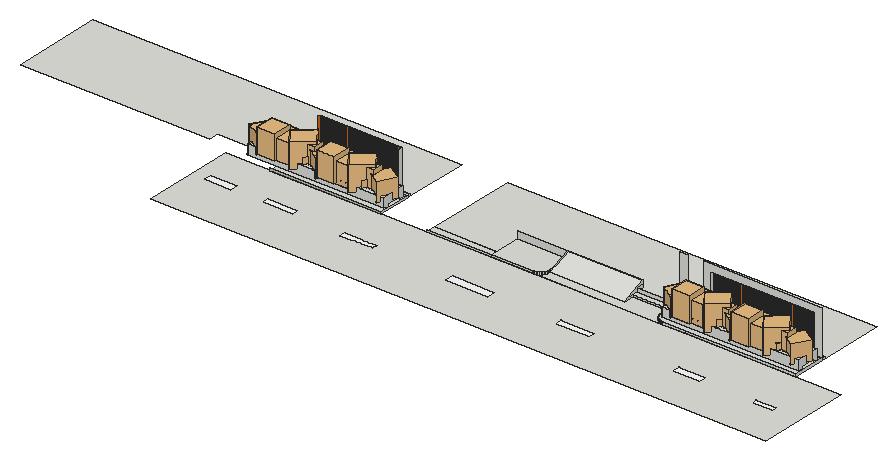
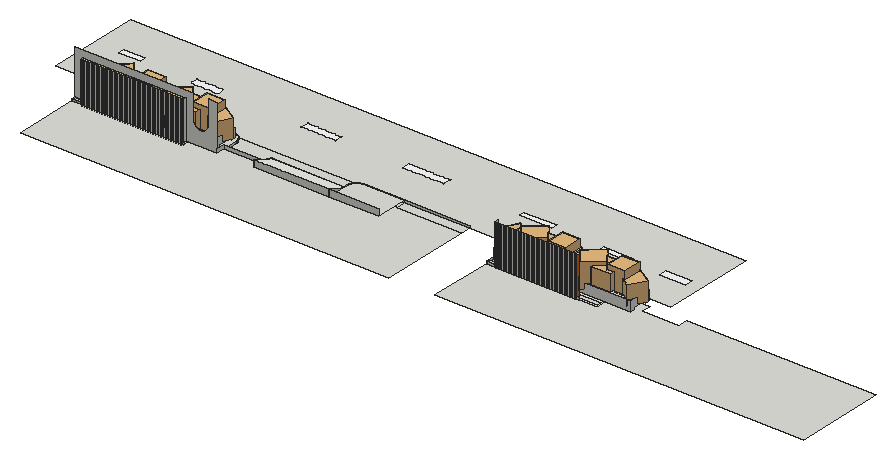
# SketchUp Ruby script. Lengths in inches.
U = 1.inch
M = Sketchup.active_model
def pt(a) = Geom::Point3d.new(a.map { |v| v * U })
def face(e, loops, mat)
  f = e.add_face(loops[0].map { |a| pt(a) })
  loops[1..].each { |l| e.add_face(l.map { |a| pt(a) }).erase! }
  f.material = f.back_material = mat if mat
  f
end
# faces: each face lists its corners as indices into pts; further lists are holes
def faces(e, pts, list, mat = nil) = list.each { |f| face(e, (f[0].is_a?(Array) ? f : [f]).map { |l| l.map { |i| pts[i] } }, mat) }
# xy, xz, yz: faces in a plane at the given z, y or x. An outline is a flat list of corners, or four numbers for a rectangle; further outlines are holes
def ring(l) = l.size == 4 ? [[l[0], l[1]], [l[2], l[1]], [l[2], l[3]], [l[0], l[3]]] : l.each_slice(2).to_a
def flat(e, list, mat, &to3) = list.each { |f| face(e, (f[0].is_a?(Array) ? f : [f]).map { |l| ring(l).map { |u, v| to3.(u, v) } }, mat) }
def xy(e, z, list, mat = nil) = flat(e, list, mat) { |x, y| [x, y, z] }
def xz(e, y, list, mat = nil) = flat(e, list, mat) { |x, z| [x, y, z] }
def yz(e, x, list, mat = nil) = flat(e, list, mat) { |y, z| [x, y, z] }
def lines(e, pts, list) = list.each { |a, b| e.add_line(pt(pts[a]), pt(pts[b])) }
# prism: a flat outline (further loops are holes) pulled along v
def prism(e, loops, v, mat = nil)
  f = face(e, loops, mat); d = Geom::Vector3d.new(v.map { |x| x * U })
  f.pushpull(f.normal.samedirection?(d) ? d.length : -d.length)
end
def box(e, o, s, mat = nil) = prism(e, [[o, [o[0] + s[0], o[1], o[2]], [o[0] + s[0], o[1] + s[1], o[2]], [o[0], o[1] + s[1], o[2]]]], [0, 0, s[2]], mat)
def at(x, y, z, deg = 0) = Geom::Transformation.translation(pt([x, y, z])) * Geom::Transformation.rotation(ORIGIN, Z_AXIS, deg.degrees)
def axes(o, x, y, z) = Geom::Transformation.new([*x, 0, *y, 0, *z, 0, *pt(o).to_a, 1])
def part(name) = M.definitions.add(name)
# library, detail: a bought-in or finely detailed component or shape, given as its bounding box
def library(name, o, s) = part(name).tap { |d| box(d.entities, o, s) }
def detail(e, o, s) = box(e.add_group.entities, o, s)
def put(e, d, t, mat = nil) = e.add_instance(d, t).tap { |i| i.material = mat if mat }
def group(e, t, mat = nil) = e.add_group.tap { |g| g.transformation = t; g.material = mat if mat }.entities
root = M.entities
M.materials.add("Color_000").color = [255, 255, 255]
M.materials.add("Material__1").color = [95, 70, 46]
M.materials.add("[0041_Chocolate]").color = [210, 105, 30]
M.materials.add("[Pavers with Grass Herringbone]").color = [197, 201, 190]
c1 = part("Untitled (5)")
xy(c1.entities,0,[[[158.81,26.5625,306.06,993.3125],[226.57,518.17,239.57,583.92],[225.28,357.51,237.28,411.51],[222.61,182.28,236.36,226.53],[239.71,931.55,251.46,972.3],[233.64,703.93,242.14,755.18],[240.05,835.03,248.8,880.53],[222.04,66.5,231.29,100.5]]])
xy(c1.entities,0,[[222.04,66.5,231.29,100.5],[222.61,182.28,236.36,226.53],[225.28,357.51,237.28,411.51],[226.57,518.17,239.57,583.92],[233.64,703.93,242.14,755.18],
  [240.05,835.03,248.8,880.53],[239.71,931.55,251.46,972.3]],"Color_000")
c2 = library("Areca palm plant",[0,0,0],[49.1,36.6,54.46])
c3 = library("Group\#74",[-84.69,-90.07,-0.36],[176.51,175.13,171.4])
c4 = library("Group20\#1",[-20.81,-17.08,3.79],[39.86,39.43,37.51])
c5 = library("Group38\#2",[14.01,28.44,-23.43],[18.58,18.32,38.89])
c6 = library("Group\#130",[-7.34,-1.2,0],[38.67,35.81,49.04])
c7 = part("Group\#8")
put(c7.entities,c2,axes([-6.2,56.6,6.08],[0.45017,-0.56191,0],[0.66137,0.52986,0],[0,0,0.72]))
put(c7.entities,c2,axes([-6.2,158.41,6.08],[0.45017,-0.56191,0],[0.66137,0.52986,0],[0,0,0.72]))
put(c7.entities,c3,axes([14.93,145.87,6.05],[-0.04961,-0.08593,0],[0.08593,-0.04961,0],[0,0,0.10522]))
put(c7.entities,c3,axes([14.93,193.18,6.05],[-0.04961,-0.08593,0],[0.08593,-0.04961,0],[0,0,0.10522]))
put(c7.entities,c4,axes([18.97,79.98,4.77],[0,0.85,0],[-0.85,0,0],[0,0,0.85]))
put(c7.entities,c3,axes([14.93,173.12,6.05],[-0.04961,-0.08593,0],[0.08593,-0.04961,0],[0,0,0.10522]))
g1 = group(c7.entities,at(0,0,0))
xy(g1,0,[[0,0,6,234.8],[30,0,36,234.8]])
xy(g1,3,[[6,0,30,234.8]])
xy(g1,7,[[6,5,30,229.8]],"Material__1")
xy(g1,15,[[[0,0,36,234.8],[6,5,30,229.8]]])
xz(g1,0,[[0,0,6,0,6,3,30,3,30,0,36,0,36,15,0,15]])
xz(g1,5,[[6,7,30,15]])
xz(g1,229.8,[[6,7,30,15]])
xz(g1,234.8,[[0,0,0,15,36,15,36,0,30,0,30,3,6,3,6,0]])
yz(g1,0,[[0,0,234.8,15]])
yz(g1,6,[[0,0,234.8,3],[5,7,229.8,15]])
yz(g1,30,[[0,0,234.8,3],[5,7,229.8,15]])
yz(g1,36,[[0,0,234.8,15]])
put(c7.entities,c3,axes([17.19,223.04,6.07],[-0.08133,-0.14087,0],[0.14087,-0.08133,0],[0,0,0.1725]))
put(c7.entities,c5,axes([-4.1,-1.15,28.17],[0.8848,0,0],[0,0.94674,0],[0,0,0.85826]))
put(c7.entities,c3,axes([17.19,15.79,6.07],[-0.08133,-0.14087,0],[0.14087,-0.08133,0],[0,0,0.1725]))
put(c7.entities,c3,axes([14.93,91.37,6.05],[-0.04961,-0.08593,0],[0.08593,-0.04961,0],[0,0,0.10522]))
put(c7.entities,c4,axes([18.97,181.79,4.77],[0,0.85,0],[-0.85,0,0],[0,0,0.85]))
put(c7.entities,c3,axes([14.93,44.05,6.05],[-0.04961,-0.08593,0],[0.08593,-0.04961,0],[0,0,0.10522]))
put(c7.entities,c6,axes([24.9375,191.72,8],[0,0.79,0],[-0.79,0,0],[0,0,0.79]))
put(c7.entities,c3,axes([17.19,121.23,6.07],[-0.08133,-0.14087,0],[0.14087,-0.08133,0],[0,0,0.1725]))
put(c7.entities,c5,axes([-4.1,100.66,28.17],[0.8848,0,0],[0,0.94674,0],[0,0,0.85826]))
put(c7.entities,c6,axes([24.9375,89.91,8],[0,0.79,0],[-0.79,0,0],[0,0,0.79]))
put(c7.entities,c3,axes([14.93,71.3,6.05],[-0.04961,-0.08593,0],[0.08593,-0.04961,0],[0,0,0.10522]))
xy(root,-8,[[1539,147.25,1713.52,162.33],[1785.21,147.25,1886.4,162.52],[1886.4,147.25,1950.69,147.25,1952.69,147.38,1954.64,147.77,1956.53,148.41,1958.33,149.3,1959.99,150.4,1961.49,151.72,1962.8,153.22,1963.91,154.88,1964.8,156.67,1965.4375,158.57,1965.83,160.52,1965.96,162.52,1886.4,162.52],[1950.69,147.25,2155.5,147.25,2153.53,147.38,2151.6,147.76,2149.73,148.4,2147.96,149.27,2146.32,150.37,2144.84,151.67,2143.53,153.15,2142.4375,154.79,2141.57,156.56,2140.93,158.43,2140.55,160.36,2140.42,162.33,2140.42,178.0625,2083.4,178.0625,2083.4,162.52,1965.96,162.52,1965.83,160.52,1965.4375,158.57,1964.8,156.67,1963.91,154.88,1962.8,153.22,1961.49,151.72,1959.99,150.4,1958.33,149.3,1956.53,148.41,1954.64,147.77,1952.69,147.38],[2155.5,147.25,2189.5,147.25,2189.5,162.33,2140.42,162.33,2140.55,160.36,2140.93,158.43,2141.57,156.56,2142.4375,154.79,2143.53,153.15,2144.84,151.67,2146.32,150.37,2147.96,149.27,2149.73,148.4,2151.6,147.76,2153.53,147.38],
  [2189.5,147.25,2364.02,162.33],[1489.92,162.33,1539,162.33,1539,203.875,1540.625,203.875,1540.625,204.875,1541.375,204.875,1541.375,203.875,1544.625,203.875,1544.625,204.875,1545.375,204.875,1545.375,203.875,1548.625,203.875,1548.625,204.875,1549.375,204.875,1549.375,203.875,1552.625,203.875,1552.625,204.875,1553.375,204.875,1553.375,203.875,1556.625,203.875,1556.625,204.875,1557.375,204.875,1557.375,203.875,1560.625,203.875,1560.625,204.875,1561.375,204.875,1561.375,203.875,1564.625,203.875,1564.625,204.875,1565.375,204.875,1565.375,203.875,1568.625,203.875,1568.625,204.875,1569.375,204.875,1569.375,203.875,1572.625,203.875,1572.625,204.875,1573.375,204.875,1573.375,203.875,1576.625,203.875,1576.625,204.875,1577.375,204.875,1577.375,203.875,1580.625,203.875,1580.625,204.875,1581.375,204.875,1581.375,203.875,1584.625,203.875,1584.625,204.875,1585.375,204.875,1585.375,203.875,1588.625,203.875,1588.625,204.875,1589.375,204.875,1589.375,203.875,1592.625,203.875,1592.625,204.875,1593.375,204.875,1593.375,203.875,1596.625,203.875,1596.625,204.875,1597.375,204.875,1597.375,203.875,1600.625,203.875,1600.625,204.875,1601.375,204.875,1601.375,203.875,1604.625,203.875,1604.625,204.875,1605.375,204.875,1605.375,203.875,1608.625,203.875,1608.625,204.875,1609.375,204.875,1609.375,203.875,1612.625,203.875,1612.625,204.875,1613.375,204.875,1613.375,203.875,1616.625,203.875,1616.625,204.875,1617.375,204.875,1617.375,203.875,1620.625,203.875,1620.625,204.875,1621.375,204.875,1621.375,203.875,1624.625,203.875,1624.625,204.875,1625.375,204.875,1625.375,203.875,1628.625,203.875,1628.625,204.875,1629.375,204.875,1629.375,203.875,1632.625,203.875,1632.625,204.875,1633.375,204.875,1633.375,203.875,1636.625,203.875,1636.625,204.875,1637.375,204.875,1637.375,203.875,1640.625,203.875,1640.625,204.875,1641.375,204.875,1641.375,203.875,1644.625,203.875,1644.625,204.875,1645.375,204.875,1645.375,203.875,1648.625,203.875,1648.625,204.875,1649.375,204.875,1649.375,203.875,1652.625,203.875,1652.625,204.875,1653.375,204.875,1653.375,203.875,1656.625,203.875,1656.625,204.875,1657.375,204.875,1657.375,203.875,1660.625,203.875,1660.625,204.875,1661.375,204.875,1661.375,203.875,1664.625,203.875,1664.625,204.875,1665.375,204.875,1665.375,203.875,1668.625,203.875,1668.625,204.875,1669.375,204.875,1669.375,203.875,1672.625,203.875,1672.625,204.875,1673.375,204.875,1673.375,203.875,1676.625,203.875,1676.625,204.875,1677.375,204.875,1677.375,203.875,1680.625,203.875,1680.625,204.875,1681.375,204.875,1681.375,203.875,1684.625,203.875,1684.625,204.875,1685.375,204.875,1685.375,203.875,1688.625,203.875,1688.625,204.875,1689.375,204.875,1689.375,203.875,1692.625,203.875,1692.625,204.875,1693.375,204.875,1693.375,203.875,1696.625,203.875,1696.625,204.875,1697.375,204.875,1697.375,203.875,1713.52,203.875,1713.52,305.58,1134.71,305.58,1134.71,162.52,1432.9,162.52,1432.9,178.0625,1489.92,178.0625],[1539,162.33,1539,203.875,1700.625,203.875,1700.625,198.625,1713.52,198.625,1713.52,162.33],[2140.42,162.33,2189.5,162.33,2189.5,203.875,2191.125,203.875,2191.125,204.875,2191.875,204.875,2191.875,203.875,2195.125,203.875,2195.125,204.875,2195.875,204.875,2195.875,203.875,2199.125,203.875,2199.125,204.875,2199.875,204.875,2199.875,203.875,2203.125,203.875,2203.125,204.875,2203.875,204.875,2203.875,203.875,2207.125,203.875,2207.125,204.875,2207.875,204.875,2207.875,203.875,2211.125,203.875,2211.125,204.875,2211.875,204.875,2211.875,203.875,2215.125,203.875,2215.125,204.875,2215.875,204.875,2215.875,203.875,2219.125,203.875,2219.125,204.875,2219.875,204.875,2219.875,203.875,2223.125,203.875,2223.125,204.875,2223.875,204.875,2223.875,203.875,2227.125,203.875,2227.125,204.875,2227.875,204.875,2227.875,203.875,2231.125,203.875,2231.125,204.875,2231.875,204.875,2231.875,203.875,2235.125,203.875,2235.125,204.875,2235.875,204.875,2235.875,203.875,2239.125,203.875,2239.125,204.875,2239.875,204.875,2239.875,203.875,2243.125,203.875,2243.125,204.875,2243.875,204.875,2243.875,203.875,2247.125,203.875,2247.125,204.875,2247.875,204.875,2247.875,203.875,2251.125,203.875,2251.125,204.875,2251.875,204.875,2251.875,203.875,2255.125,203.875,2255.125,204.875,2255.875,204.875,2255.875,203.875,2259.125,203.875,2259.125,204.875,2259.875,204.875,2259.875,203.875,2263.125,203.875,2263.125,204.875,2263.875,204.875,2263.875,203.875,2267.125,203.875,2267.125,204.875,2267.875,204.875,2267.875,203.875,2271.125,203.875,2271.125,204.875,2271.875,204.875,2271.875,203.875,2275.125,203.875,2275.125,204.875,2275.875,204.875,2275.875,203.875,2279.125,203.875,2279.125,204.875,2279.875,204.875,2279.875,203.875,2283.125,203.875,2283.125,204.875,2283.875,204.875,2283.875,203.875,2287.125,203.875,2287.125,204.875,2287.875,204.875,2287.875,203.875,2291.125,203.875,2291.125,204.875,2291.875,204.875,2291.875,203.875,2295.125,203.875,2295.125,204.875,2295.875,204.875,2295.875,203.875,2299.125,203.875,2299.125,204.875,2299.875,204.875,2299.875,203.875,2303.125,203.875,2303.125,204.875,2303.875,204.875,2303.875,203.875,2307.125,203.875,2307.125,204.875,2307.875,204.875,2307.875,203.875,2311.125,203.875,2311.125,204.875,2311.875,204.875,2311.875,203.875,2315.125,203.875,2315.125,204.875,2315.875,204.875,2315.875,203.875,2319.125,203.875,2319.125,204.875,2319.875,204.875,2319.875,203.875,2323.125,203.875,2323.125,204.875,2323.875,204.875,2323.875,203.875,2327.125,203.875,2327.125,204.875,2327.875,204.875,2327.875,203.875,2331.125,203.875,2331.125,204.875,2331.875,204.875,2331.875,203.875,2335.125,203.875,2335.125,204.875,2335.875,204.875,2335.875,203.875,2339.125,203.875,2339.125,204.875,2339.875,204.875,2339.875,203.875,2343.125,203.875,2343.125,204.875,2343.875,204.875,2343.875,203.875,2347.125,203.875,2347.125,204.875,2347.875,204.875,2347.875,203.875,2364.02,203.875,2364.02,305.58,1785.21,305.58,1785.21,162.52,2083.4,162.52,2083.4,178.0625,2140.42,178.0625],[2189.5,162.33,2189.5,203.875,2351.125,203.875,2351.125,198.625,2364.02,198.625,2364.02,162.33],
  [1700.625,198.625,1713.52,203.875],[2351.125,198.625,2364.02,203.875]])
xy(root,-4.67,[[1886.4,147.25,1950.69,147.25,1952.69,147.38,1954.64,147.77,1956.53,148.41,1958.33,149.3,1959.99,150.4,1961.49,151.72,1962.8,153.22,1963.91,154.88,1964.8,156.67,1965.4375,158.57,1965.83,160.52,1965.96,162.52,1965.96,198.625,1886.4,198.625],[2155.5,147.25,2364.02,147.25,2364.02,198.625,2140.42,198.625,2140.42,162.33,2140.55,160.36,2140.93,158.43,2141.57,156.56,2142.4375,154.79,2143.53,153.15,2144.84,151.67,2146.32,150.37,2147.96,149.27,2149.73,148.4,2151.6,147.76,2153.53,147.38],[2083.4,178.0625,2140.42,185.9375],[1539,198.625,1713.52,203.875],[2189.5,198.625,2364.02,203.875]])
xz(root,147.25,[[1785.21,-8,1886.4,-4.67],[1886.4,-8,1950.69,-4.67],[2155.5,-8,2189.5,-4.67],[2189.5,-8,2364.02,-4.67]])
xz(root,147.25,[[1539,-8,1713.52,-4.67]],"[Pavers with Grass Herringbone]")
xz(root,178.0625,[[2083.4,-8,2140.42,-4.67]])
xz(root,185.9375,[[2083.4,-4.67,2140.42,0.73]])
xz(root,198.625,[[1700.625,-8,1713.52,-4.67],[2351.125,-8,2364.02,-4.67],[1886.4,-4.67,1965.96,6.125],[1965.96,-4.67,2083.4,6.125],[2140.42,-4.67,2189.5,-4.67,2189.5,55.1875,2351.125,55.1875,2351.125,-4.67,2364.02,-4.67,2364.02,66.125,2178.1,66.125,2178.1,26.79,2177.21,24.11,2175.74,21.71,2173.77,19.69,2171.4,18.17,2168.74,17.23,2165.94,16.91,2163.14,17.23,2160.49,18.17,2158.11,19.69,2156.14,21.71,2154.67,24.11,2153.79,26.79,2153.79,66.125,2140.66,66.125,2140.66,6.125,2140.42,6.125]])
xz(root,203.875,[[1569.375,-8,1572.625,-4.67],[1572.625,-8,1573.375,-4.67],[1573.375,-8,1576.625,-4.67],[1576.625,-8,1577.375,-4.67],[1577.375,-8,1580.625,-4.67],
  [1580.625,-8,1581.375,-4.67],[1581.375,-8,1584.625,-4.67],[1584.625,-8,1585.375,-4.67],[1585.375,-8,1588.625,-4.67],[1588.625,-8,1589.375,-4.67],
  [1589.375,-8,1592.625,-4.67],[1592.625,-8,1593.375,-4.67],[1593.375,-8,1596.625,-4.67],[1596.625,-8,1597.375,-4.67],[1597.375,-8,1600.625,-4.67],
  [1600.625,-8,1601.375,-4.67],[1601.375,-8,1604.625,-4.67],[1604.625,-8,1605.375,-4.67],[1605.375,-8,1608.625,-4.67],[1608.625,-8,1609.375,-4.67],
  [1609.375,-8,1612.625,-4.67],[1612.625,-8,1613.375,-4.67],[1613.375,-8,1616.625,-4.67],[1616.625,-8,1617.375,-4.67],[1617.375,-8,1620.625,-4.67],
  [1620.625,-8,1621.375,-4.67],[1621.375,-8,1624.625,-4.67],[1624.625,-8,1625.375,-4.67],[1625.375,-8,1628.625,-4.67],[1628.625,-8,1629.375,-4.67],
  [1629.375,-8,1632.625,-4.67],[1632.625,-8,1633.375,-4.67],[1633.375,-8,1636.625,-4.67],[1636.625,-8,1637.375,-4.67],[1637.375,-8,1640.625,-4.67],
  [1640.625,-8,1641.375,-4.67],[1641.375,-8,1644.625,-4.67],[1644.625,-8,1645.375,-4.67],[1645.375,-8,1648.625,-4.67],[1648.625,-8,1649.375,-4.67],
  [1649.375,-8,1652.625,-4.67],[1652.625,-8,1653.375,-4.67],[1653.375,-8,1656.625,-4.67],[1656.625,-8,1657.375,-4.67],[1657.375,-8,1660.625,-4.67],
  [1660.625,-8,1661.375,-4.67],[1661.375,-8,1664.625,-4.67],[1664.625,-8,1665.375,-4.67],[1665.375,-8,1668.625,-4.67],[1668.625,-8,1669.375,-4.67],
  [1669.375,-8,1672.625,-4.67],[1672.625,-8,1673.375,-4.67],[1673.375,-8,1676.625,-4.67],[1676.625,-8,1677.375,-4.67],[1677.375,-8,1680.625,-4.67],
  [1680.625,-8,1681.375,-4.67],[1681.375,-8,1684.625,-4.67],[1684.625,-8,1685.375,-4.67],[1685.375,-8,1688.625,-4.67],[1688.625,-8,1689.375,-4.67],
  [1689.375,-8,1692.625,-4.67],[1692.625,-8,1693.375,-4.67],[1693.375,-8,1696.625,-4.67],[1696.625,-8,1697.375,-4.67],[1697.375,-8,1700.625,-4.67],
  [1700.625,-8,1713.52,-4.67],[2189.5,-8,2191.125,-4.67],[2191.125,-8,2191.875,-4.67],[2191.875,-8,2195.125,-4.67],[2195.125,-8,2195.875,-4.67],
  [2195.875,-8,2199.125,-4.67],[2199.125,-8,2199.875,-4.67],[2199.875,-8,2203.125,-4.67],[2203.125,-8,2203.875,-4.67],[2203.875,-8,2207.125,-4.67],
  [2207.125,-8,2207.875,-4.67],[2207.875,-8,2211.125,-4.67],[2211.125,-8,2211.875,-4.67],[2211.875,-8,2215.125,-4.67],[2215.125,-8,2215.875,-4.67],
  [2215.875,-8,2219.125,-4.67],[2219.125,-8,2219.875,-4.67],[2219.875,-8,2223.125,-4.67],[2223.125,-8,2223.875,-4.67],[2223.875,-8,2227.125,-4.67],
  [2227.125,-8,2227.875,-4.67],[2227.875,-8,2231.125,-4.67],[2231.125,-8,2231.875,-4.67],[2231.875,-8,2235.125,-4.67],[2235.125,-8,2235.875,-4.67],
  [2235.875,-8,2239.125,-4.67],[2239.125,-8,2239.875,-4.67],[2239.875,-8,2243.125,-4.67],[2243.125,-8,2243.875,-4.67],[2243.875,-8,2247.125,-4.67],
  [2247.125,-8,2247.875,-4.67],[2247.875,-8,2251.125,-4.67],[2251.125,-8,2251.875,-4.67],[2251.875,-8,2255.125,-4.67],[2255.125,-8,2255.875,-4.67],
  [2255.875,-8,2259.125,-4.67],[2259.125,-8,2259.875,-4.67],[2259.875,-8,2263.125,-4.67],[2263.125,-8,2263.875,-4.67],[2263.875,-8,2267.125,-4.67],
  [2267.125,-8,2267.875,-4.67],[2267.875,-8,2271.125,-4.67],[2271.125,-8,2271.875,-4.67],[2271.875,-8,2275.125,-4.67],[2275.125,-8,2275.875,-4.67],
  [2275.875,-8,2279.125,-4.67],[2279.125,-8,2279.875,-4.67],[2279.875,-8,2283.125,-4.67],[2283.125,-8,2283.875,-4.67],[2283.875,-8,2287.125,-4.67],
  [2287.125,-8,2287.875,-4.67],[2287.875,-8,2291.125,-4.67],[2291.125,-8,2291.875,-4.67],[2291.875,-8,2295.125,-4.67],[2295.125,-8,2295.875,-4.67],
  [2295.875,-8,2299.125,-4.67],[2299.125,-8,2299.875,-4.67],[2299.875,-8,2303.125,-4.67],[2303.125,-8,2303.875,-4.67],[2303.875,-8,2307.125,-4.67],
  [2307.125,-8,2307.875,-4.67],[2307.875,-8,2311.125,-4.67],[2311.125,-8,2311.875,-4.67],[2311.875,-8,2315.125,-4.67],[2315.125,-8,2315.875,-4.67],
  [2315.875,-8,2319.125,-4.67],[2319.125,-8,2319.875,-4.67],[2319.875,-8,2323.125,-4.67],[2323.125,-8,2323.875,-4.67],[2323.875,-8,2327.125,-4.67],
  [2327.125,-8,2327.875,-4.67],[2327.875,-8,2331.125,-4.67],[2331.125,-8,2331.875,-4.67],[2331.875,-8,2335.125,-4.67],[2335.125,-8,2335.875,-4.67],
  [2335.875,-8,2339.125,-4.67],[2339.125,-8,2339.875,-4.67],[2339.875,-8,2343.125,-4.67],[2343.125,-8,2343.875,-4.67],[2343.875,-8,2347.125,-4.67],
  [2347.125,-8,2347.875,-4.67],[2347.875,-8,2351.125,-4.67],[2351.125,-8,2364.02,-4.67]])
xz(root,203.875,[[1569.375,-4.67,1572.625,55.1875],[1573.375,-4.67,1576.625,55.1875],[1577.375,-4.67,1580.625,55.1875],[1581.375,-4.67,1584.625,55.1875],[1585.375,-4.67,1588.625,55.1875],
  [1589.375,-4.67,1592.625,55.1875],[1593.375,-4.67,1596.625,55.1875],[1597.375,-4.67,1600.625,55.1875],[1601.375,-4.67,1604.625,55.1875],[1605.375,-4.67,1608.625,55.1875],
  [1609.375,-4.67,1612.625,55.1875],[1613.375,-4.67,1616.625,55.1875],[1617.375,-4.67,1620.625,55.1875],[1621.375,-4.67,1624.625,55.1875],[1625.375,-4.67,1628.625,55.1875],
  [1629.375,-4.67,1632.625,55.1875],[1633.375,-4.67,1636.625,55.1875],[1637.375,-4.67,1640.625,55.1875],[1641.375,-4.67,1644.625,55.1875],[1645.375,-4.67,1648.625,55.1875],
  [1649.375,-4.67,1652.625,55.1875],[1653.375,-4.67,1656.625,55.1875],[1657.375,-4.67,1660.625,55.1875],[1661.375,-4.67,1664.625,55.1875],[1665.375,-4.67,1668.625,55.1875],
  [1669.375,-4.67,1672.625,55.1875],[1673.375,-4.67,1676.625,55.1875],[1677.375,-4.67,1680.625,55.1875],[1681.375,-4.67,1684.625,55.1875],[1685.375,-4.67,1688.625,55.1875],
  [1689.375,-4.67,1692.625,55.1875],[1693.375,-4.67,1696.625,55.1875],[1697.375,-4.67,1700.625,55.1875],[2189.5,-4.67,2191.125,55.1875],[2191.875,-4.67,2195.125,55.1875],
  [2195.875,-4.67,2199.125,55.1875],[2199.875,-4.67,2203.125,55.1875],[2203.875,-4.67,2207.125,55.1875],[2207.875,-4.67,2211.125,55.1875],[2211.875,-4.67,2215.125,55.1875],
  [2215.875,-4.67,2219.125,55.1875],[2219.875,-4.67,2223.125,55.1875],[2223.875,-4.67,2227.125,55.1875],[2227.875,-4.67,2231.125,55.1875],[2231.875,-4.67,2235.125,55.1875],
  [2235.875,-4.67,2239.125,55.1875],[2239.875,-4.67,2243.125,55.1875],[2243.875,-4.67,2247.125,55.1875],[2247.875,-4.67,2251.125,55.1875],[2251.875,-4.67,2255.125,55.1875],
  [2255.875,-4.67,2259.125,55.1875],[2259.875,-4.67,2263.125,55.1875],[2263.875,-4.67,2267.125,55.1875],[2267.875,-4.67,2271.125,55.1875],[2271.875,-4.67,2275.125,55.1875],
  [2275.875,-4.67,2279.125,55.1875],[2279.875,-4.67,2283.125,55.1875],[2283.875,-4.67,2287.125,55.1875],[2287.875,-4.67,2291.125,55.1875],[2291.875,-4.67,2295.125,55.1875],
  [2295.875,-4.67,2299.125,55.1875],[2299.875,-4.67,2303.125,55.1875],[2303.875,-4.67,2307.125,55.1875],[2307.875,-4.67,2311.125,55.1875],[2311.875,-4.67,2315.125,55.1875],
  [2315.875,-4.67,2319.125,55.1875],[2319.875,-4.67,2323.125,55.1875],[2323.875,-4.67,2327.125,55.1875],[2327.875,-4.67,2331.125,55.1875],[2331.875,-4.67,2335.125,55.1875],
  [2335.875,-4.67,2339.125,55.1875],[2339.875,-4.67,2343.125,55.1875],[2343.875,-4.67,2347.125,55.1875],[2347.875,-4.67,2351.125,55.1875]],"[0041_Chocolate]")
xz(root,204.875,[[1572.625,-8,1573.375,55.1875],[1576.625,-8,1577.375,55.1875],[1580.625,-8,1581.375,55.1875],[1584.625,-8,1585.375,55.1875],[1588.625,-8,1589.375,55.1875],
  [1592.625,-8,1593.375,55.1875],[1596.625,-8,1597.375,55.1875],[1600.625,-8,1601.375,55.1875],[1604.625,-8,1605.375,55.1875],[1608.625,-8,1609.375,55.1875],
  [1612.625,-8,1613.375,55.1875],[1616.625,-8,1617.375,55.1875],[1620.625,-8,1621.375,55.1875],[1624.625,-8,1625.375,55.1875],[1628.625,-8,1629.375,55.1875],
  [1632.625,-8,1633.375,55.1875],[1636.625,-8,1637.375,55.1875],[1640.625,-8,1641.375,55.1875],[1644.625,-8,1645.375,55.1875],[1648.625,-8,1649.375,55.1875],
  [1652.625,-8,1653.375,55.1875],[1656.625,-8,1657.375,55.1875],[1660.625,-8,1661.375,55.1875],[1664.625,-8,1665.375,55.1875],[1668.625,-8,1669.375,55.1875],
  [1672.625,-8,1673.375,55.1875],[1676.625,-8,1677.375,55.1875],[1680.625,-8,1681.375,55.1875],[1684.625,-8,1685.375,55.1875],[1688.625,-8,1689.375,55.1875],
  [1692.625,-8,1693.375,55.1875],[1696.625,-8,1697.375,55.1875],[2191.125,-8,2191.875,55.1875],[2195.125,-8,2195.875,55.1875],[2199.125,-8,2199.875,55.1875],
  [2203.125,-8,2203.875,55.1875],[2207.125,-8,2207.875,55.1875],[2211.125,-8,2211.875,55.1875]])
yz(root,1572.625,[[203.875,-8,204.875,55.1875]])
yz(root,1573.375,[[203.875,-8,204.875,55.1875]])
yz(root,1576.625,[[203.875,-8,204.875,55.1875]])
yz(root,1577.375,[[203.875,-8,204.875,55.1875]])
yz(root,1580.625,[[203.875,-8,204.875,55.1875]])
yz(root,1581.375,[[203.875,-8,204.875,55.1875]])
yz(root,1584.625,[[203.875,-8,204.875,55.1875]])
yz(root,1585.375,[[203.875,-8,204.875,55.1875]])
yz(root,1588.625,[[203.875,-8,204.875,55.1875]])
yz(root,1589.375,[[203.875,-8,204.875,55.1875]])
yz(root,1592.625,[[203.875,-8,204.875,55.1875]])
yz(root,1593.375,[[203.875,-8,204.875,55.1875]])
yz(root,1596.625,[[203.875,-8,204.875,55.1875]])
yz(root,1597.375,[[203.875,-8,204.875,55.1875]])
yz(root,1600.625,[[203.875,-8,204.875,55.1875]])
yz(root,1601.375,[[203.875,-8,204.875,55.1875]])
yz(root,1604.625,[[203.875,-8,204.875,55.1875]])
yz(root,1605.375,[[203.875,-8,204.875,55.1875]])
yz(root,1608.625,[[203.875,-8,204.875,55.1875]])
yz(root,1609.375,[[203.875,-8,204.875,55.1875]])
yz(root,1612.625,[[203.875,-8,204.875,55.1875]])
yz(root,1613.375,[[203.875,-8,204.875,55.1875]])
yz(root,1616.625,[[203.875,-8,204.875,55.1875]])
yz(root,1617.375,[[203.875,-8,204.875,55.1875]])
yz(root,1620.625,[[203.875,-8,204.875,55.1875]])
yz(root,1621.375,[[203.875,-8,204.875,55.1875]])
yz(root,1624.625,[[203.875,-8,204.875,55.1875]])
yz(root,1625.375,[[203.875,-8,204.875,55.1875]])
yz(root,1628.625,[[203.875,-8,204.875,55.1875]])
yz(root,1629.375,[[203.875,-8,204.875,55.1875]])
yz(root,1632.625,[[203.875,-8,204.875,55.1875]])
yz(root,1633.375,[[203.875,-8,204.875,55.1875]])
yz(root,1636.625,[[203.875,-8,204.875,55.1875]])
yz(root,1637.375,[[203.875,-8,204.875,55.1875]])
yz(root,1640.625,[[203.875,-8,204.875,55.1875]])
yz(root,1641.375,[[203.875,-8,204.875,55.1875]])
yz(root,1644.625,[[203.875,-8,204.875,55.1875]])
yz(root,1645.375,[[203.875,-8,204.875,55.1875]])
yz(root,1648.625,[[203.875,-8,204.875,55.1875]])
yz(root,1649.375,[[203.875,-8,204.875,55.1875]])
yz(root,1652.625,[[203.875,-8,204.875,55.1875]])
yz(root,1653.375,[[203.875,-8,204.875,55.1875]])
yz(root,1656.625,[[203.875,-8,204.875,55.1875]])
yz(root,1657.375,[[203.875,-8,204.875,55.1875]])
yz(root,1660.625,[[203.875,-8,204.875,55.1875]])
yz(root,1661.375,[[203.875,-8,204.875,55.1875]])
yz(root,1664.625,[[203.875,-8,204.875,55.1875]])
yz(root,1665.375,[[203.875,-8,204.875,55.1875]])
yz(root,1668.625,[[203.875,-8,204.875,55.1875]])
yz(root,1669.375,[[203.875,-8,204.875,55.1875]])
yz(root,1672.625,[[203.875,-8,204.875,55.1875]])
yz(root,1673.375,[[203.875,-8,204.875,55.1875]])
yz(root,1676.625,[[203.875,-8,204.875,55.1875]])
yz(root,1677.375,[[203.875,-8,204.875,55.1875]])
yz(root,1680.625,[[203.875,-8,204.875,55.1875]])
yz(root,1681.375,[[203.875,-8,204.875,55.1875]])
yz(root,1684.625,[[203.875,-8,204.875,55.1875]])
yz(root,1685.375,[[203.875,-8,204.875,55.1875]])
yz(root,1688.625,[[203.875,-8,204.875,55.1875]])
yz(root,1689.375,[[203.875,-8,204.875,55.1875]])
yz(root,1692.625,[[203.875,-8,204.875,55.1875]])
yz(root,1693.375,[[203.875,-8,204.875,55.1875]])
yz(root,1696.625,[[203.875,-8,204.875,55.1875]])
yz(root,1697.375,[[203.875,-8,204.875,55.1875]])
yz(root,1700.625,[[198.625,-8,203.875,55.1875]])
yz(root,1713.52,[[147.25,-8,198.625,-4.67],[198.625,-8,203.875,-4.67]])
yz(root,1965.96,[[162.52,-8,171.04,-4.67,162.52,-4.67],[171.04,-4.67,198.625,6.125,198.625,-4.67]])
yz(root,2083.4,[[162.52,-8,178.0625,-8,178.0625,-4.67,171.04,-4.67],[171.04,-4.67,185.9375,-4.67,185.9375,0.73,198.625,0.73,198.625,6.125],[185.9375,-4.67,198.625,0.73]])
yz(root,2140.42,[[162.33,-8,178.0625,-4.67],[185.9375,-4.67,198.625,0.73]])
yz(root,2189.5,[[198.625,-4.67,203.875,55.1875]])
yz(root,2191.125,[[203.875,-8,204.875,55.1875]])
yz(root,2191.875,[[203.875,-8,204.875,55.1875]])
yz(root,2195.125,[[203.875,-8,204.875,55.1875]])
yz(root,2195.875,[[203.875,-8,204.875,55.1875]])
yz(root,2199.125,[[203.875,-8,204.875,55.1875]])
yz(root,2199.875,[[203.875,-8,204.875,55.1875]])
yz(root,2203.125,[[203.875,-8,204.875,55.1875]])
yz(root,2203.875,[[203.875,-8,204.875,55.1875]])
yz(root,2207.125,[[203.875,-8,204.875,55.1875]])
yz(root,2207.875,[[203.875,-8,204.875,55.1875]])
yz(root,2211.125,[[203.875,-8,204.875,55.1875]])
yz(root,2211.875,[[203.875,-8,204.875,55.1875]])
yz(root,2215.125,[[203.875,-8,204.875,55.1875]])
yz(root,2215.875,[[203.875,-8,204.875,55.1875]])
yz(root,2219.125,[[203.875,-8,204.875,55.1875]])
yz(root,2219.875,[[203.875,-8,204.875,55.1875]])
yz(root,2223.125,[[203.875,-8,204.875,55.1875]])
yz(root,2223.875,[[203.875,-8,204.875,55.1875]])
yz(root,2227.125,[[203.875,-8,204.875,55.1875]])
yz(root,2227.875,[[203.875,-8,204.875,55.1875]])
yz(root,2231.125,[[203.875,-8,204.875,55.1875]])
yz(root,2231.875,[[203.875,-8,204.875,55.1875]])
yz(root,2235.125,[[203.875,-8,204.875,55.1875]])
yz(root,2235.875,[[203.875,-8,204.875,55.1875]])
yz(root,2239.125,[[203.875,-8,204.875,55.1875]])
yz(root,2239.875,[[203.875,-8,204.875,55.1875]])
yz(root,2243.125,[[203.875,-8,204.875,55.1875]])
yz(root,2243.875,[[203.875,-8,204.875,55.1875]])
yz(root,2247.125,[[203.875,-8,204.875,55.1875]])
yz(root,2247.875,[[203.875,-8,204.875,55.1875]])
yz(root,2251.125,[[203.875,-8,204.875,55.1875]])
yz(root,2251.875,[[203.875,-8,204.875,55.1875]])
yz(root,2255.125,[[203.875,-8,204.875,55.1875]])
yz(root,2255.875,[[203.875,-8,204.875,55.1875]])
yz(root,2259.125,[[203.875,-8,204.875,55.1875]])
yz(root,2259.875,[[203.875,-8,204.875,55.1875]])
yz(root,2263.125,[[203.875,-8,204.875,55.1875]])
yz(root,2263.875,[[203.875,-8,204.875,55.1875]])
yz(root,2267.125,[[203.875,-8,204.875,55.1875]])
yz(root,2267.875,[[203.875,-8,204.875,55.1875]])
yz(root,2271.125,[[203.875,-8,204.875,55.1875]])
yz(root,2271.875,[[203.875,-8,204.875,55.1875]])
yz(root,2275.125,[[203.875,-8,204.875,55.1875]])
yz(root,2275.875,[[203.875,-8,204.875,55.1875]])
yz(root,2279.125,[[203.875,-8,204.875,55.1875]])
yz(root,2279.875,[[203.875,-8,204.875,55.1875]])
yz(root,2283.125,[[203.875,-8,204.875,55.1875]])
yz(root,2283.875,[[203.875,-8,204.875,55.1875]])
yz(root,2287.125,[[203.875,-8,204.875,55.1875]])
yz(root,2287.875,[[203.875,-8,204.875,55.1875]])
yz(root,2291.125,[[203.875,-8,204.875,55.1875]])
yz(root,2291.875,[[203.875,-8,204.875,55.1875]])
yz(root,2295.125,[[203.875,-8,204.875,55.1875]])
yz(root,2295.875,[[203.875,-8,204.875,55.1875]])
yz(root,2299.125,[[203.875,-8,204.875,55.1875]])
yz(root,2299.875,[[203.875,-8,204.875,55.1875]])
yz(root,2303.125,[[203.875,-8,204.875,55.1875]])
yz(root,2303.875,[[203.875,-8,204.875,55.1875]])
yz(root,2307.125,[[203.875,-8,204.875,55.1875]])
yz(root,2307.875,[[203.875,-8,204.875,55.1875]])
yz(root,2311.125,[[203.875,-8,204.875,55.1875]])
yz(root,2311.875,[[203.875,-8,204.875,55.1875]])
yz(root,2315.125,[[203.875,-8,204.875,55.1875]])
yz(root,2315.875,[[203.875,-8,204.875,55.1875]])
yz(root,2319.125,[[203.875,-8,204.875,55.1875]])
yz(root,2319.875,[[203.875,-8,204.875,55.1875]])
yz(root,2323.125,[[203.875,-8,204.875,55.1875]])
yz(root,2323.875,[[203.875,-8,204.875,55.1875]])
yz(root,2327.125,[[203.875,-8,204.875,55.1875]])
yz(root,2327.875,[[203.875,-8,204.875,55.1875]])
yz(root,2331.125,[[203.875,-8,204.875,55.1875]])
yz(root,2331.875,[[203.875,-8,204.875,55.1875]])
yz(root,2335.125,[[203.875,-8,204.875,55.1875]])
yz(root,2335.875,[[203.875,-8,204.875,55.1875]])
yz(root,2339.125,[[203.875,-8,204.875,55.1875]])
yz(root,2339.875,[[203.875,-8,204.875,55.1875]])
yz(root,2343.125,[[203.875,-8,204.875,55.1875]])
yz(root,2343.875,[[203.875,-8,204.875,55.1875]])
yz(root,2347.125,[[203.875,-8,204.875,55.1875]])
yz(root,2347.875,[[203.875,-8,204.875,55.1875]])
yz(root,2351.125,[[198.625,-8,203.875,55.1875]])
yz(root,2364.02,[[147.25,-8,198.625,-4.67],[198.625,-8,203.875,-4.67]])
p = [[1952.69,147.38,-4.67],[1950.69,147.25,-4.67],[1950.69,147.25,-8],[1952.69,147.38,-8],[2155.5,147.25,-4.67],[2153.53,147.38,-4.67],
  [2153.53,147.38,-8],[2155.5,147.25,-8],[1954.64,147.77,-4.67],[1954.64,147.77,-8],[2151.6,147.76,-4.67],[2151.6,147.76,-8],
  [1956.53,148.41,-4.67],[1956.53,148.41,-8],[2149.73,148.4,-4.67],[2149.73,148.4,-8],[1958.33,149.3,-4.67],[1958.33,149.3,-8],
  [2147.96,149.27,-4.67],[2147.96,149.27,-8],[1959.99,150.4,-4.67],[1959.99,150.4,-8],[2146.32,150.37,-4.67],[2146.32,150.37,-8],
  [1961.49,151.72,-4.67],[1961.49,151.72,-8],[2144.84,151.67,-4.67],[2144.84,151.67,-8],[1962.8,153.22,-4.67],[1962.8,153.22,-8],
  [2143.53,153.15,-4.67],[2143.53,153.15,-8],[1963.91,154.88,-4.67],[1963.91,154.88,-8],[2142.4375,154.79,-4.67],[2142.4375,154.79,-8],
  [2141.57,156.56,-4.67],[2141.57,156.56,-8],[1964.8,156.67,-4.67],[1964.8,156.67,-8],[2140.93,158.43,-4.67],[2140.93,158.43,-8],
  [1965.4375,158.57,-4.67],[1965.4375,158.57,-8],[2140.55,160.36,-4.67],[2140.55,160.36,-8],[1965.83,160.52,-4.67],[1965.83,160.52,-8],
  [2140.42,162.33,-4.67],[2140.42,162.33,-8],[1965.96,162.52,-4.67],[1965.96,162.52,-8],[2083.4,162.52,-8],[2083.4,171.04,-4.67],
  [2083.4,198.625,6.125],[1965.96,198.625,6.125],[1965.96,171.04,-4.67]]
faces(root,p,[[0,1,2,3],[4,5,6,7],[8,0,3,9],[5,10,11,6],[12,8,9,13],[10,14,15,11],[16,12,13,17],[14,18,19,15],
  [20,16,17,21],[18,22,23,19],[24,20,21,25],[22,26,27,23],[28,24,25,29],[26,30,31,27],[32,28,29,33],[30,34,35,31],
  [34,36,37,35],[38,32,33,39],[36,40,41,37],[42,38,39,43],[40,44,45,41],[46,42,43,47],[44,48,49,45],[50,46,47,51],
  [52,53,54,55,56,51]])
put(root,c1,at(2462.27,-158.81,-8.49,90))
put(root,c7,axes([1711.06,156.31,-4.73],[0,1,0],[-0.9127,0,0],[0,0,1]))
put(root,c7,axes([2361.56,156.31,-4.73],[0,1,0],[-0.9127,0,0],[0,0,1]))
